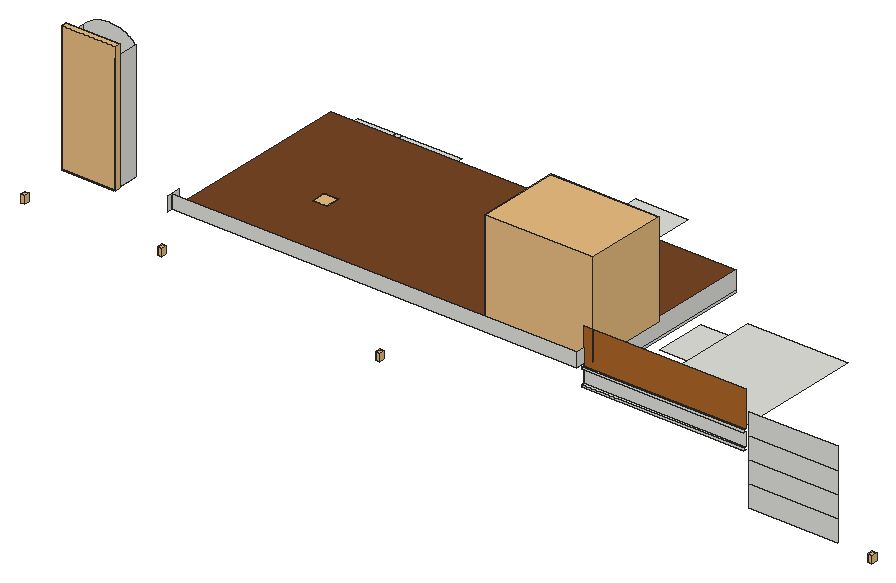
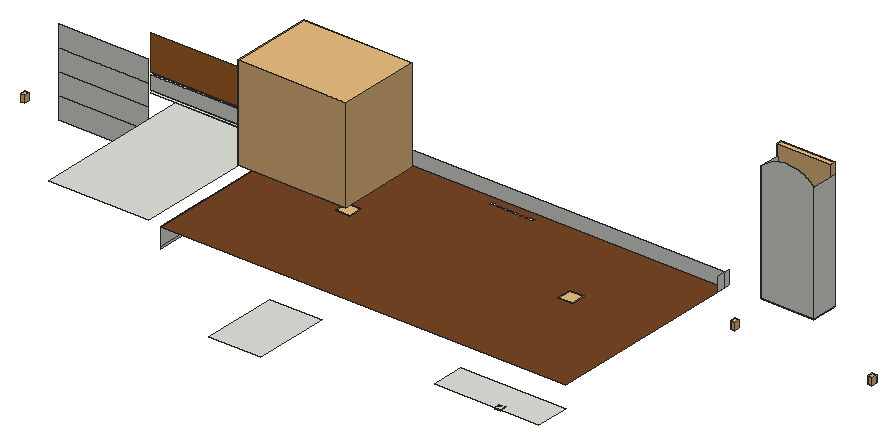
# SketchUp Ruby script. Lengths in inches.
U = 1.inch
M = Sketchup.active_model
def pt(a) = Geom::Point3d.new(a.map { |v| v * U })
def face(e, loops, mat)
  f = e.add_face(loops[0].map { |a| pt(a) })
  loops[1..].each { |l| e.add_face(l.map { |a| pt(a) }).erase! }
  f.material = f.back_material = mat if mat
  f
end
# faces: each face lists its corners as indices into pts; further lists are holes
def faces(e, pts, list, mat = nil) = list.each { |f| face(e, (f[0].is_a?(Array) ? f : [f]).map { |l| l.map { |i| pts[i] } }, mat) }
# xy, xz, yz: faces in a plane at the given z, y or x. An outline is a flat list of corners, or four numbers for a rectangle; further outlines are holes
def ring(l) = l.size == 4 ? [[l[0], l[1]], [l[2], l[1]], [l[2], l[3]], [l[0], l[3]]] : l.each_slice(2).to_a
def flat(e, list, mat, &to3) = list.each { |f| face(e, (f[0].is_a?(Array) ? f : [f]).map { |l| ring(l).map { |u, v| to3.(u, v) } }, mat) }
def xy(e, z, list, mat = nil) = flat(e, list, mat) { |x, y| [x, y, z] }
def xz(e, y, list, mat = nil) = flat(e, list, mat) { |x, z| [x, y, z] }
def yz(e, x, list, mat = nil) = flat(e, list, mat) { |y, z| [x, y, z] }
def lines(e, pts, list) = list.each { |a, b| e.add_line(pt(pts[a]), pt(pts[b])) }
# prism: a flat outline (further loops are holes) pulled along v
def prism(e, loops, v, mat = nil)
  f = face(e, loops, mat); d = Geom::Vector3d.new(v.map { |x| x * U })
  f.pushpull(f.normal.samedirection?(d) ? d.length : -d.length)
end
def box(e, o, s, mat = nil) = prism(e, [[o, [o[0] + s[0], o[1], o[2]], [o[0] + s[0], o[1] + s[1], o[2]], [o[0], o[1] + s[1], o[2]]]], [0, 0, s[2]], mat)
def at(x, y, z, deg = 0) = Geom::Transformation.translation(pt([x, y, z])) * Geom::Transformation.rotation(ORIGIN, Z_AXIS, deg.degrees)
def axes(o, x, y, z) = Geom::Transformation.new([*x, 0, *y, 0, *z, 0, *pt(o).to_a, 1])
def part(name) = M.definitions.add(name)
# library, detail: a bought-in or finely detailed component or shape, given as its bounding box
def library(name, o, s) = part(name).tap { |d| box(d.entities, o, s) }
def detail(e, o, s) = box(e.add_group.entities, o, s)
def put(e, d, t, mat = nil) = e.add_instance(d, t).tap { |i| i.material = mat if mat }
def group(e, t, mat = nil) = e.add_group.tap { |g| g.transformation = t; g.material = mat if mat }.entities
root = M.entities
M.materials.add("[Wood Bamboo]").color = [173, 103, 41]
M.materials.add("[Wood Veneer 01]").color = [120, 70, 37]
c1 = library("Lamp Wall Outdoor 94-02",[-1.89,-4.65,-3.17],[3.78,4.65,6.35])
c2 = part("Copyright 2018, ")
xy(c2.entities,0.05,[[[19.06,0,19.06,9.82,21.3125,9.82,22.13,9.76,22.85,9.6,23.48,9.33,24,8.95,24.43,8.48,24.73,7.92,24.91,7.28,24.97,6.54,24.91,5.85,24.74,5.21,24.46,4.64,24.0625,4.14,23.58,3.73,23.03,3.4375,22.42,3.26,21.75,3.2,21.1,3.27,20.375,3.48,20.375,0],[21.62,4.3125,22.05,4.35,22.4375,4.47,22.79,4.66,23.09,4.94,23.34,5.28,23.52,5.66,23.63,6.09,23.67,6.56,23.6,7.16,23.4,7.68,23.08,8.1,22.66,8.39,22.08,8.56,21.28,8.61,20.375,8.61,20.375,4.61,20.98,4.39]],[25.77,0,27.98,4.71,25.47,9.82,26.9375,9.82,28.69,6.14,30.375,9.82,31.82,9.82,27.21,0],[[43.77,0,43.11,0.03,42.52,0.14,41.99,0.3125,41.54,0.55,41.18,0.86,40.92,1.2,40.77,1.6,40.71,2.04,40.82,2.64,41.12,3.13,41.63,3.5,42.35,3.75,41.86,4.16,41.74,4.37,41.7,4.57,41.77,4.87,41.98,5.14,42.3,5.36,42.73,5.51,42.1,5.88,41.65,6.34,41.38,6.91,41.29,7.57,41.34,8.0625,41.48,8.5,41.72,8.88,42.05,9.21,42.47,9.48,42.95,9.67,43.5,9.78,44.13,9.82,46.81,9.82,46.81,8.8125,45.49,8.8125,46.02,8.11,46.13,7.77,46.17,7.38,46.1,6.875,45.88,6.38,45.55,5.94,45.13,5.625,44.53,5.39,43.64,5.21,43.09,5.03,42.96,4.89,42.91,4.71,42.98,4.5,43.18,4.34,44.17,4.04,45.71,3.625,46.33,3.2,46.67,2.67,46.79,2.03,46.74,1.59,46.59,1.2,46.33,0.85,45.97,0.55,45.52,0.31,45.01,0.14,44.42,0.03],[43.74,1.02,44.5,1.09,45.0625,1.28,45.42,1.58,45.53,1.99,45.5,2.2,45.39,2.4,44.94,2.72,44.26,2.9375,43.41,3.01,42.82,2.94,42.34,2.73,42.03,2.42,41.93,2.03,42.04,1.59,42.38,1.28,42.95,1.09],[43.72,6.34,44.22,6.42,44.63,6.67,44.91,7.05,45,7.51,44.9,7.98,44.63,8.36,44.22,8.61,43.71,8.7,43.23,8.61,42.82,8.35,42.54,7.96,42.45,7.5,42.54,7.04,42.8125,6.67,43.22,6.42]],[180.16,0,182.36,4.71,179.85,9.82,181.32,9.82,183.07,6.14,184.75,9.82,186.2,9.82,181.59,0],[[219.8,0,219.13,0.03,218.54,0.14,218.02,0.3125,217.57,0.55,217.21,0.86,216.95,1.2,216.79,1.6,216.74,2.04,216.84,2.64,217.15,3.13,217.66,3.5,218.375,3.75,217.89,4.16,217.77,4.37,217.72,4.57,217.79,4.87,218,5.14,218.33,5.36,218.76,5.51,218.13,5.88,217.68,6.34,217.41,6.91,217.32,7.57,217.37,8.0625,217.51,8.5,217.75,8.88,218.08,9.21,218.5,9.48,218.98,9.67,219.53,9.78,220.16,9.82,222.83,9.82,222.83,8.8125,221.52,8.8125,222.05,8.11,222.16,7.77,222.2,7.38,222.125,6.875,221.91,6.38,221.58,5.94,221.16,5.625,220.5625,5.39,219.67,5.21,219.12,5.03,218.99,4.89,218.94,4.71,219.01,4.5,219.21,4.34,220.2,4.04,221.73,3.625,222.35,3.2,222.7,2.67,222.82,2.03,222.77,1.59,222.61,1.2,222.36,0.85,222,0.55,221.55,0.31,221.03,0.14,220.45,0.03],[219.77,1.02,220.53,1.09,221.09,1.28,221.44,1.58,221.5625,1.99,221.52,2.2,221.41,2.4,220.97,2.72,220.29,2.9375,219.43,3.01,218.84,2.94,218.37,2.73,218.0625,2.42,217.96,2.03,218.07,1.59,218.41,1.28,218.98,1.09],[219.75,6.34,220.25,6.42,220.66,6.67,220.93,7.05,221.02,7.51,220.93,7.98,220.66,8.36,220.24,8.61,219.74,8.7,219.25,8.61,218.85,8.35,218.57,7.96,218.48,7.5,218.57,7.04,218.84,6.67,219.25,6.42]],
  [92.62,1.6,92.62,1.87,92.89,2.17,93.07,2.48,93.22,3.3125,92.89,3.45,92.65,3.66,92.51,3.92,92.47,4.24,92.53,4.6,92.72,4.9,93.01,5.11,93.34,5.18,93.73,5.08,94.04,4.8,94.25,4.36,94.32,3.82,94.2,3.09,93.87,2.45,93.33,1.9375],[6.01,3.2,5.21,3.24,4.48,3.37,3.81,3.58,3.2,3.87,2.66,4.23,2.17,4.66,1.74,5.14,1.38,5.7,1.08,6.29,0.875,6.91,0.75,7.55,0.71,8.22,0.8,9.25,1.09,10.2,1.57,11.07,2.24,11.84,3.06,12.49,3.96,12.95,4.95,13.22,6.04,13.3125,6.83,13.26,7.68,13.11,8.5625,12.86,9.49,12.5,9.49,10.98,8.63,11.42,7.78,11.72,6.9375,11.91,6.11,11.97,5.29,11.9,4.55,11.7,3.89,11.37,3.29,10.9,2.8,10.33,2.45,9.7,2.24,8.99,2.17,8.22,2.24,7.44,2.45,6.74,2.79,6.11,3.27,5.55,3.86,5.09,4.53,4.76,5.27,4.57,6.09,4.5,6.98,4.57,7.87,4.78,8.74,5.12,9.6,5.6,9.6,4.05,8.79,3.68,7.92,3.41,6.99,3.25],[[14.21,3.2,13.51,3.26,12.87,3.4375,12.29,3.73,11.77,4.14,11.34,4.65,11.03,5.21,10.85,5.82,10.78,6.5,10.85,7.1875,11.03,7.81,11.34,8.375,11.78,8.88,12.31,9.3,12.9,9.59,13.55,9.77,14.27,9.83,14.98,9.77,15.63,9.59,16.21,9.29,16.73,8.87,17.16,8.36,17.47,7.79,17.66,7.16,17.72,6.47,17.66,5.79,17.47,5.18,17.16,4.625,16.72,4.13,16.19,3.72,15.6,3.43,14.9375,3.26],[14.25,4.4,14.71,4.44,15.12,4.55,15.48,4.74,15.81,5,16.07,5.32,16.26,5.68,16.37,6.08,16.41,6.53,16.37,6.97,16.25,7.375,16.06,7.74,15.78,8.0625,15.45,8.33,15.07,8.52,14.65,8.63,14.2,8.67,13.76,8.63,13.36,8.52,13,8.33,12.68,8.0625,12.42,7.74,12.23,7.37,12.12,6.97,12.08,6.52,12.12,6.07,12.24,5.67,12.43,5.31,12.69,4.99,13.02,4.73,13.39,4.55,13.8,4.44]],[57.3125,3.2,56.51,3.33,55.84,3.72,55.54,4.07,55.34,4.58,55.26,5.77,55.26,8.66,54.13,8.66,54.13,8.78,56.54,11.16,56.54,9.82,58.6,9.82,58.6,8.66,56.54,8.66,56.54,5.48,56.6,4.99,56.78,4.64,57.06,4.43,57.47,4.36,58.18,4.48,58.93,4.82,58.93,3.62,58.16,3.31],[[88.3125,3.2,87.67,3.25,87.08,3.41,86.54,3.66,86.06,4.02,85.66,4.45,85.37,4.93,85.2,5.46,85.14,6.04,85.23,6.75,85.49,7.37,85.93,7.91,86.54,8.36,86,8.86,85.64,9.37,85.4375,9.91,85.37,10.54,85.43,11.1,85.59,11.61,85.86,12.08,86.24,12.51,86.7,12.86,87.21,13.11,87.76,13.26,88.37,13.3125,88.96,13.26,89.51,13.11,90.01,12.86,90.46,12.51,90.83,12.09,91.09,11.62,91.25,11.1,91.31,10.54,91.23,9.91,91,9.33,90.62,8.82,90.08,8.36,90.68,7.91,91.11,7.38,91.36,6.75,91.45,6.02,91.39,5.4375,91.23,4.91,90.95,4.43,90.56,4,90.08,3.65,89.55,3.4,88.96,3.25],[88.33,4.54,89,4.64,89.54,4.94,89.9,5.39,90.02,5.96,90.02,6.11,89.9,6.72,89.54,7.21,88.98,7.53,88.28,7.64,87.6,7.53,87.05,7.21,86.69,6.71,86.57,6.09,86.69,5.47,87.06,4.98,87.62,4.65],[88.35,9.02,88.95,9.125,89.45,9.45,89.79,9.93,89.9,10.49,89.79,11.08,89.46,11.55,88.96,11.87,88.34,11.97,87.72,11.87,87.22,11.5625,86.89,11.09,86.78,10.51,86.89,9.9375,87.24,9.46,87.75,9.13]],
  [[113.29,3.2,112.92,3.24,112.64,3.36,112.43,3.57,112.32,3.85,111.9,3.57,111.47,3.375,111.03,3.26,110.57,3.22,109.95,3.33,109.44,3.66,109.1,4.17,108.99,4.79,109.1,5.375,109.43,5.89,109.97,6.32,110.6875,6.66,112.33,7.22,112.33,7.57,112.26,8.08,112.04,8.45,111.67,8.67,111.16,8.74,110.64,8.67,110.12,8.47,109.61,8.13,109.11,7.65,109.11,9.06,109.53,9.45,110.02,9.72,110.6,9.89,111.27,9.94,111.77,9.91,112.21,9.81,112.61,9.63,112.95,9.39,113.34,8.92,113.55,8.34,113.6,7.22,113.6,4.46,113.65,4.21,113.82,4.13,114.12,4.21,114.55,4.47,114.55,3.6875,113.85,3.3],[111.19,4.1,111.79,4.22,112.33,4.6,112.33,6.53,111.47,6.2,110.91,5.9375,110.54,5.67,110.34,5.375,110.27,5.01,110.33,4.64,110.53,4.35,110.82,4.16]],[121.02,3.2,120.43,3.28,119.88,3.51,119.43,3.87,119.1,4.34,118.9,5.04,118.83,6.09,118.83,9.82,120.12,9.82,120.12,6.11,120.19,5.24,120.41,4.68,120.82,4.38,121.44,4.28,121.88,4.33,122.29,4.5,122.66,4.78,123,5.17,123,9.82,124.29,9.82,124.29,3.3125,123,3.3125,123,4.15,122.5625,3.75,122.07,3.45,121.54,3.26],[[156.36,3.2,155.99,3.24,155.7,3.36,155.5,3.57,155.39,3.85,154.97,3.57,154.54,3.375,154.1,3.26,153.64,3.22,153.02,3.33,152.51,3.66,152.17,4.17,152.06,4.79,152.17,5.375,152.5,5.89,153.03,6.32,153.75,6.66,155.4,7.22,155.4,7.57,155.33,8.08,155.11,8.45,154.74,8.67,154.23,8.74,153.7,8.67,153.1875,8.47,152.68,8.13,152.18,7.65,152.18,9.06,152.59,9.45,153.09,9.72,153.67,9.89,154.33,9.94,154.83,9.91,155.28,9.81,155.68,9.63,156.02,9.39,156.4,8.92,156.62,8.34,156.66,7.22,156.66,4.46,156.72,4.21,156.89,4.13,157.1875,4.21,157.62,4.47,157.62,3.6875,156.92,3.3],[154.26,4.1,154.85,4.22,155.4,4.6,155.4,6.53,154.54,6.2,153.98,5.9375,153.61,5.67,153.4,5.375,153.34,5.01,153.4,4.64,153.59,4.35,153.89,4.16]],[161.74,3.2,161.01,3.26,160.37,3.43,159.8,3.71,159.3,4.11,158.91,4.6,158.62,5.16,158.45,5.81,158.4,6.53,158.45,7.26,158.62,7.92,158.89,8.5,159.28,9,159.76,9.41,160.3,9.71,160.92,9.88,161.6,9.94,162.51,9.85,163.49,9.49,163.49,8.12,162.55,8.59,161.68,8.74,161.27,8.7,160.89,8.59,160.55,8.4,160.25,8.13,160.01,7.8,159.84,7.4375,159.73,7.02,159.7,6.57,159.73,6.1,159.85,5.68,160.04,5.31,160.3,4.99,160.63,4.73,161.01,4.55,161.44,4.4375,161.93,4.4,162.73,4.51,163.63,4.83,163.63,3.5625,162.67,3.29],[[178.37,3.2,178,3.24,177.71,3.36,177.51,3.57,177.39,3.85,176.98,3.57,176.55,3.375,176.1,3.26,175.65,3.22,175.02,3.33,174.52,3.66,174.18,4.17,174.0625,4.79,174.17,5.375,174.51,5.89,175.04,6.32,175.76,6.66,177.41,7.22,177.41,7.57,177.33,8.08,177.11,8.45,176.75,8.67,176.23,8.74,175.71,8.67,175.19,8.47,174.6875,8.13,174.18,7.65,174.18,9.06,174.6,9.45,175.1,9.72,175.68,9.89,176.34,9.94,176.84,9.91,177.29,9.81,177.68,9.63,178.03,9.39,178.41,8.92,178.625,8.34,178.67,7.22,178.67,4.46,178.73,4.21,178.9,4.13,179.2,4.21,179.625,4.47,179.625,3.6875,178.92,3.3],[176.27,4.1,176.86,4.22,177.41,4.6,177.41,6.53,176.54,6.2,175.98,5.9375,175.61,5.67,175.41,5.375,175.34,5.01,175.41,4.64,175.6,4.35,175.9,4.16]],
  [210.76,3.2,209.73,3.33,208.59,3.78,208.59,5.17,209.71,4.55,210.23,4.37,210.66,4.3125,211.04,4.36,211.36,4.51,211.57,4.73,211.65,4.98,211.6,5.24,211.46,5.45,210.65,5.99,209.62,6.64,209.02,7.18,208.73,7.69,208.64,8.25,208.67,8.6,208.78,8.93,208.96,9.22,209.22,9.47,209.89,9.83,210.72,9.94,211.6875,9.81,212.68,9.41,212.68,8.13,211.64,8.65,210.81,8.83,210.47,8.79,210.2,8.67,210.03,8.48,209.97,8.25,210.02,8.03,210.18,7.82,210.91,7.32,211.37,7.06,212.08,6.59,212.59,6.09,212.89,5.57,213,5.02,212.96,4.64,212.84,4.3,212.64,3.99,212.37,3.71,212.04,3.49,211.66,3.33],[[73.82,3.22,73.14,3.3,72.53,3.56,71.99,3.99,71.52,4.59,71.14,5.34,70.87,6.2,70.7,7.17,70.65,8.25,70.71,9.32,70.875,10.29,71.16,11.15,71.55,11.9,72.03,12.52,72.58,12.96,73.2,13.23,73.88,13.3125,74.53,13.23,75.12,12.96,75.65,12.51,76.125,11.89,76.51,11.13,76.79,10.27,76.96,9.32,77.01,8.28,76.96,7.2,76.79,6.24,76.51,5.38,76.125,4.62,75.65,4.01,75.11,3.57,74.5,3.3],[73.81,4.52,74.2,4.58,74.54,4.77,74.84,5.08,75.1,5.51,75.31,6.06,75.46,6.6875,75.58,8.22,75.46,9.76,75.32,10.4,75.12,10.95,74.87,11.4,74.59,11.72,74.26,11.91,73.89,11.97,73.82,11.97,73.4375,11.91,73.09,11.72,72.79,11.41,72.53,10.97,72.32,10.43,72.18,9.79,72.06,8.26,72.17,6.7,72.32,6.06,72.52,5.51,72.78,5.08,73.08,4.77,73.42,4.58]],[[204.86,3.22,203.89,3.33,203.125,3.66,202.53,4.18,202.06,4.86,201.76,5.67,201.66,6.6,201.71,7.31,201.87,7.95,202.13,8.51,202.5,9.01,202.95,9.42,203.47,9.71,204.05,9.89,204.6875,9.94,205.3,9.89,205.85,9.72,206.33,9.43,206.75,9.04,207.09,8.55,207.33,7.98,207.47,7.34,207.52,6.61,207.52,6.45,202.95,6.45,203.13,5.61,203.32,5.27,203.57,4.97,203.88,4.73,204.23,4.55,205.06,4.42,205.68,4.47,206.28,4.61,206.86,4.86,207.41,5.21,207.41,3.95,206.82,3.61,206.23,3.39,205.6,3.26],[202.98,7.22,206.25,7.22,206.11,7.9,205.79,8.41,205.31,8.72,204.6875,8.83,204.06,8.72,203.55,8.41,203.1875,7.9]],[32.81,3.3125,32.81,9.82,34.1,9.82,34.1,8.33,34.17,8.4375,34.64,9.1,35.1,9.57,35.57,9.85,36.04,9.94,36.4,9.9,36.78,9.76,37.55,9.21,36.875,8.08,36.23,8.55,35.63,8.71,35.33,8.68,35.05,8.57,34.55,8.12,34.21,7.47,34.1,6.71,34.1,3.3125],[38.48,3.3125,39.77,9.82],
  [47.77,3.3125,47.77,13.1875,49.06,13.1875,49.06,8.96,49.49,9.39,49.96,9.7,50.49,9.88,51.06,9.94,51.68,9.86,52.23,9.62,52.68,9.23,52.99,8.72,53.18,8.01,53.24,7.02,53.24,3.3125,51.96,3.3125,51.96,7.34,51.87,7.98,51.61,8.48,51.2,8.81,50.6875,8.92,50.27,8.86,49.89,8.7,49.49,8.41,49.06,7.97,49.06,3.3125],[63.46,3.3125,63.46,3.41,64.06,4.11,66.27,7.04,66.95,8.09,67.35,8.86,67.53,9.47,67.6,10.07,67.48,10.82,67.125,11.41,66.57,11.79,65.87,11.92,65.28,11.83,64.7,11.57,64.15,11.14,63.66,10.58,63.66,12.375,64.24,12.79,64.83,13.08,65.43,13.26,66.04,13.3125,66.65,13.26,67.21,13.1,67.72,12.83,68.17,12.45,68.53,11.99,68.79,11.47,68.95,10.9,69,10.26,68.95,9.65,68.8,8.99,68.51,8.27,68.06,7.4375,67.34,6.4,66.26,5.04,65.95,4.68,69.71,4.68,69.71,3.3125],[80.37,3.3125,81.78,13.1875],[100.21,3.3125,100.21,13.1875,101.625,13.1875,101.625,8.67,105.78,13.1875,107.55,13.1875,103.27,8.5,108.6,3.3125,106.67,3.3125,101.625,8.19,101.625,3.3125],[115.72,3.3125,117,13.1875],
  [126.04,3.3125,126.04,9.82,127.33,9.82,127.33,8.96,127.82,9.39,128.3,9.7,128.78,9.88,129.25,9.94,129.83,9.87,130.35,9.65,130.79,9.28,131.17,8.77,131.6875,9.29,132.22,9.66,132.77,9.88,133.32,9.96,133.77,9.91,134.18,9.78,134.55,9.57,134.88,9.27,135.15,8.875,135.34,8.39,135.45,7.82,135.49,7.15,135.49,3.3125,134.2,3.3125,134.2,7.17,134.12,7.88,133.87,8.41,133.47,8.73,132.92,8.84,132.53,8.79,132.15,8.64,131.78,8.39,131.43,8.04,131.43,3.3125,130.13,3.3125,130.13,6.93,130.0625,7.85,129.84,8.44,129.67,8.63,129.45,8.76,128.83,8.87,128.45,8.82,128.1,8.6875,127.74,8.43,127.33,8.04,127.33,3.3125],[141.43,3.3125,141.43,13.1875,142.77,13.1875,146.05,9.13,149.31,13.1875,150.63,13.1875,150.63,3.3125,149.21,3.3125,149.21,11,146.17,7.18,145.91,7.18,142.84,11,142.84,3.3125],[165.29,3.3125,165.29,13.1875,166.7,13.1875,166.7,8.67,170.86,13.1875,172.62,13.1875,168.34,8.5,173.67,3.3125,171.75,3.3125,166.7,8.19,166.7,3.3125],[214.51,3.3125,215.8,9.82],[223.8,3.3125,223.8,9.82,225.12,9.82,225.12,8.99,225.5625,9.41,226.04,9.7,226.54,9.88,227.07,9.94,227.66,9.86,228.2,9.63,228.67,9.26,229,8.77,229.2,8.06,229.27,7.03,229.27,3.3125,227.99,3.3125,227.99,7.02,227.91,7.87,227.68,8.44,227.28,8.76,226.66,8.87,226.23,8.8125,225.82,8.64,225.45,8.36,225.12,7.96,225.12,3.3125],
  [[191.3125,3.33,191.3125,13.1875,194.64,13.1875,195.6,13.15,196.45,13.04,197.19,12.85,197.83,12.58,198.39,12.25,198.88,11.84,199.32,11.36,199.7,10.81,200,10.21,200.22,9.58,200.35,8.93,200.39,8.25,200.29,7.28,200.01,6.35,199.54,5.5,198.92,4.76,198.14,4.14,197.24,3.7,196.22,3.4,194.4375,3.33],[192.73,4.59,194.54,4.59,195.48,4.62,196.18,4.73,197.16,5.1,197.88,5.65,198.34,6.21,198.66,6.85,198.86,7.55,198.93,8.33,198.86,9.08,198.66,9.77,198.32,10.38,197.85,10.92,197.43,11.26,196.94,11.53,195.97,11.85,194.49,11.93,192.73,11.93]],[39.12,11.03,38.84,11.09,38.59,11.26,38.42,11.51,38.37,11.8,38.42,12.08,38.59,12.32,38.84,12.49,39.12,12.55,39.41,12.5,39.66,12.33,39.83,12.09,39.89,11.8,39.83,11.51,39.66,11.26,39.41,11.09],[215.14,11.03,214.87,11.09,214.62,11.26,214.45,11.51,214.4,11.8,214.45,12.08,214.62,12.32,214.87,12.49,215.14,12.55,215.44,12.5,215.6875,12.33,215.86,12.09,215.92,11.8,215.86,11.51,215.6875,11.26,215.44,11.09]])
c3 = library("Spot Light",[-8.21,-8.21,-2.75],[16.42,16.42,2.75])
c4 = library("Tlon Light 1950 Ceiling 152 010",[-38.39,-38.39,-3.78],[76.78,76.78,3.41])
c5 = library("Rectangular Planter with Plant",[-49.93,-33.04,0],[93.24,71.01,81.08])
c6 = library("Group\#13",[0,0,0],[46.48,4.68,111.63])
xy(root,206.83,[[973.0625,998.1875,1001.875,1042.875]])
xy(root,209.35,[[834.07,1080.1875,878.82,1146.3125]])
xy(root,214.23,[[1005.21,916.1875,1091.46,1053.125]])
xy(root,214.57,[[624.25,1080.1875,714.02,1109]])
xy(root,215.04,[[973.0625,914.15,1112.75,916.1875]])
xy(root,217.04,[[973.0625,914.15,1112.75,916.1875]])
xy(root,228.78,[[973.0625,914.15,1112.75,916.1875]])
xy(root,230.78,[[973.0625,914.15,1112.75,916.1875]])
xy(root,232.51,[[782.66,915.1875,782.66,917.0625,820.03,917.0625,820.03,915.1875,817.03,915.1875,817.03,916.1875,785.84,916.1875,785.84,915.1875]])
xy(root,232.51,[[[624.25,908.5,973.0625,1080.1875],[782.66,915.1875,785.84,915.1875,785.84,916.1875,817.03,916.1875,817.03,915.1875,820.03,915.1875,820.03,917.0625,782.66,917.0625]]],"[Wood Veneer 01]")
xy(root,240.28,[[541.1875,893.4375,586.375,916.1875]])
xy(root,241.08,[[541.1875,893.4375,587,916.1875]])
xz(root,893.4375,[[541.1875,240.28,586.375,241.08]])
xz(root,908.5,[[624.25,232.51,973.0625,244.51]])
xz(root,914.15,[[973.0625,215.04,1112.75,217.04],[973.0625,228.78,1112.75,230.78]])
xz(root,916.1875,[[973.0625,217.04,1112.75,228.78],[541.1875,241.08,587,241.08,587,342.64,586.375,342.64,585.26,343.76,584.0625,344.84,582.81,345.86,581.5,346.82,580.15,347.7,578.75,348.51,577.3125,349.24,575.84,349.9,574.33,350.49,572.8,350.99,571.24,351.41,569.66,351.75,568.06,352,566.45,352.18,564.84,352.26,563.22,352.27,561.61,352.18,560,352.02,558.41,351.77,556.82,351.43,555.26,351.02,553.73,350.52,552.22,349.95,550.74,349.29,549.3,348.5625,547.9,347.76,546.54,346.88,545.23,345.93,543.97,344.92,542.77,343.84,541.625,342.7,541.1875,342.21]])
xz(root,916.1875,[[973.0625,230.78,1112.75,261.47]],"[Wood Bamboo]")
xz(root,919.75,[[1112.75,168.31,1189.1875,186.91],[1112.75,186.91,1189.1875,205.51],[1112.75,205.51,1189.1875,224.11],[1112.75,224.11,1189.1875,242.71]])
yz(root,541.1875,[[893.4375,241.08,916.1875,342.21]])
yz(root,587,[[893.4375,241.08,916.1875,342.64]])
yz(root,624.25,[[904.1875,232.51,908.5,244.51],[908.5,232.51,916.1875,244.51]])
yz(root,973.0625,[[914.15,215.04,1080.1875,217.04],[916.1875,217.04,916.1875,228.78,914.15,228.78,914.15,230.78,916.1875,230.78,916.1875,232.51,1080.1875,232.51,1080.1875,217.04],[908.5,232.51,916.1875,244.51]])
put(root,c1,at(1223.66,916.1875,171.53))
put(root,c1,at(799.21,916.1875,178.51))
put(root,c1,at(502.52,904.1875,201.38))
put(root,c1,at(620.92,904.1875,202.36))
put(root,c2,axes([872.05,1084.14,207.85],[-0.13928,0,0],[0,-0.1494,0],[0,0,0.93236]))
put(root,c3,axes([659.8125,1106.375,214.57],[0.32,0,0],[0,0.32,0],[0,0,0.32]))
put(root,c4,axes([696.92,983.24,232.57],[0.16,0,0],[0,0.16,0],[0,0,0.16]))
put(root,c4,axes([889.17,983.24,232.57],[0.16,0,0],[0,0.16,0],[0,0,0.16]))
put(root,c5,at(937.65,949.23,236.28))
put(root,c6,at(541.1875,893.4375,240.28))
